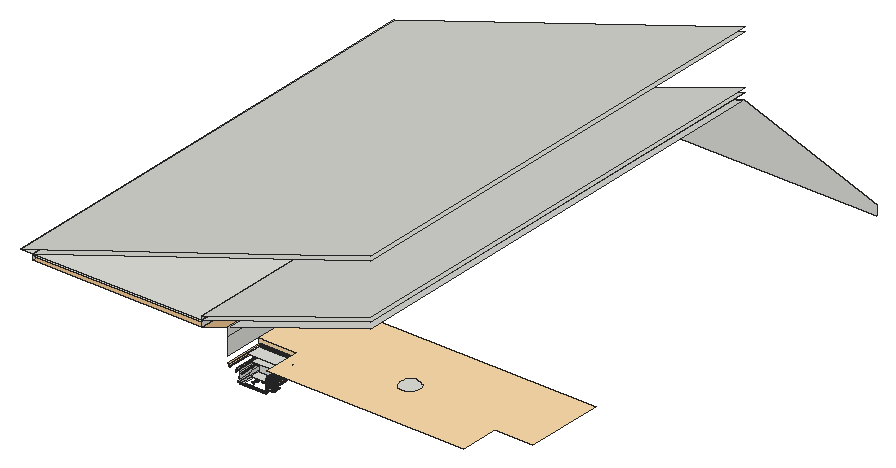
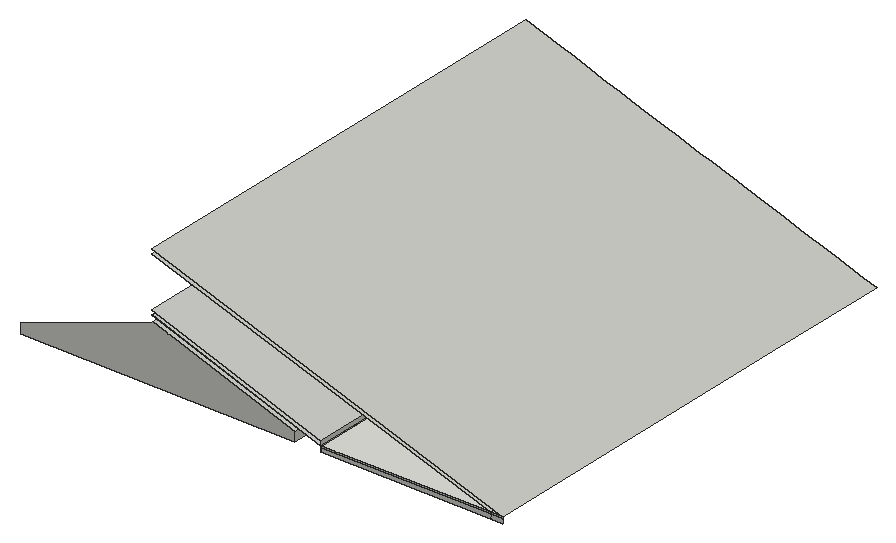
# SketchUp Ruby script. Lengths in inches.
U = 1.inch
M = Sketchup.active_model
def pt(a) = Geom::Point3d.new(a.map { |v| v * U })
def face(e, loops, mat)
  f = e.add_face(loops[0].map { |a| pt(a) })
  loops[1..].each { |l| e.add_face(l.map { |a| pt(a) }).erase! }
  f.material = f.back_material = mat if mat
  f
end
# faces: each face lists its corners as indices into pts; further lists are holes
def faces(e, pts, list, mat = nil) = list.each { |f| face(e, (f[0].is_a?(Array) ? f : [f]).map { |l| l.map { |i| pts[i] } }, mat) }
# xy, xz, yz: faces in a plane at the given z, y or x. An outline is a flat list of corners, or four numbers for a rectangle; further outlines are holes
def ring(l) = l.size == 4 ? [[l[0], l[1]], [l[2], l[1]], [l[2], l[3]], [l[0], l[3]]] : l.each_slice(2).to_a
def flat(e, list, mat, &to3) = list.each { |f| face(e, (f[0].is_a?(Array) ? f : [f]).map { |l| ring(l).map { |u, v| to3.(u, v) } }, mat) }
def xy(e, z, list, mat = nil) = flat(e, list, mat) { |x, y| [x, y, z] }
def xz(e, y, list, mat = nil) = flat(e, list, mat) { |x, z| [x, y, z] }
def yz(e, x, list, mat = nil) = flat(e, list, mat) { |y, z| [x, y, z] }
def lines(e, pts, list) = list.each { |a, b| e.add_line(pt(pts[a]), pt(pts[b])) }
# prism: a flat outline (further loops are holes) pulled along v
def prism(e, loops, v, mat = nil)
  f = face(e, loops, mat); d = Geom::Vector3d.new(v.map { |x| x * U })
  f.pushpull(f.normal.samedirection?(d) ? d.length : -d.length)
end
def box(e, o, s, mat = nil) = prism(e, [[o, [o[0] + s[0], o[1], o[2]], [o[0] + s[0], o[1] + s[1], o[2]], [o[0], o[1] + s[1], o[2]]]], [0, 0, s[2]], mat)
def at(x, y, z, deg = 0) = Geom::Transformation.translation(pt([x, y, z])) * Geom::Transformation.rotation(ORIGIN, Z_AXIS, deg.degrees)
def axes(o, x, y, z) = Geom::Transformation.new([*x, 0, *y, 0, *z, 0, *pt(o).to_a, 1])
def part(name) = M.definitions.add(name)
# library, detail: a bought-in or finely detailed component or shape, given as its bounding box
def library(name, o, s) = part(name).tap { |d| box(d.entities, o, s) }
def detail(e, o, s) = box(e.add_group.entities, o, s)
def put(e, d, t, mat = nil) = e.add_instance(d, t).tap { |i| i.material = mat if mat }
def group(e, t, mat = nil) = e.add_group.tap { |g| g.transformation = t; g.material = mat if mat }.entities
root = M.entities
M.materials.add("[0033_NavajoWhite]").color = [255, 222, 173]
M.materials.add("[0036_BurlyWood]").color = [222, 184, 135]
xy(root,94.95,[[[110.21,8.1,123.2,21.09],[111,9.67,122.41,19.51]]])
xy(root,95.99,[[110.21,14.59,123.2,21.09]])
xy(root,95.99,[[[109.69,7.58,123.72,21.61],[109.86,7.74,123.55,21.44]]],"[0033_NavajoWhite]")
xy(root,102.72,[[109.03,22.27,108.83,22.47,124.58,22.47,124.38,22.27]])
xy(root,102.72,[[108.83,22.47,108.04,23.25,125.37,23.25,124.58,22.47]],"[0033_NavajoWhite]")
xy(root,102.86,[[111,14.59,122.41,19.51]])
xy(root,105.42,[[108.83,14.59,124.58,22.47]])
xy(root,108.125,[[178.61,26.68,177.27,26.85,176.02,27.37,174.95,28.2,174.12,29.27,173.6,30.52,173.43,31.86,173.6,33.21,174.12,34.46,174.95,35.53,176.02,36.36,177.27,36.875,178.61,37.05,179.96,36.875,181.21,36.36,182.28,35.53,183.11,34.46,183.625,33.21,183.8,31.86,183.625,30.52,183.11,29.27,182.28,28.2,181.21,27.37,179.96,26.85]])
xy(root,108.125,[[[126.55,4.75,126.55,24.44,106.86,24.44,106.86,64.75,247.8,64.75,247.8,24.44,228.12,24.44,228.12,4.75],[178.61,26.68,179.96,26.85,181.21,27.37,182.28,28.2,183.11,29.27,183.625,30.52,183.8,31.86,183.625,33.21,183.11,34.46,182.28,35.53,181.21,36.36,179.96,36.875,178.61,37.05,177.27,36.875,176.02,36.36,174.95,35.53,174.12,34.46,173.6,33.21,173.43,31.86,173.6,30.52,174.12,29.27,174.95,28.2,176.02,27.37,177.27,26.85]]],"[0033_NavajoWhite]")
xy(root,117,[[6.32,4.75,93.16,64.75],[93.16,4.75,93.71,64.75]],"[0036_BurlyWood]")
xy(root,119,[[6.32,4.75,93.16,244.75]])
xy(root,120,[[0,4.75,6.32,64.75],[6.32,4.75,93.16,244.75],[0,64.75,6.32,244.75]])
xz(root,19.51,[[111,94.95,122.41,102.86]])
xz(root,21.09,[[110.21,94.95,123.2,95.1],[110.21,95.1,123.2,95.99],[110.21,95.99,123.2,97.5625],[110.21,97.5625,123.2,99.87],[110.21,99.87,123.2,100.56],
  [110.21,100.56,123.2,101.46]])
xz(root,21.61,[[109.69,95.99,123.72,96.66]])
xz(root,22.47,[[108.83,102.72,124.58,105.42]])
xz(root,24.44,[[106.86,105.42,126.55,108.125]],"[0033_NavajoWhite]")
xz(root,64.75,[[155.99,93.75,191.99,96],[93.71,117,106.86,117,106.86,121.52]])
xz(root,244.75,[[0,117,6.32,119],[6.32,117,93.16,119],[106.86,117,106.86,121.52,179.96,146.625,247.8,122.125,247.8,117],[0,119,6.32,120],[6.32,119,93.16,120]])
yz(root,6.32,[[4.75,117,64.75,119],[4.75,119,64.75,120],[64.75,119,244.75,120]])
yz(root,93.16,[[4.75,117,244.75,119],[4.75,119,244.75,119.98],[4.75,119.98,244.75,120],[4.75,120,244.75,122.1]])
yz(root,106.86,[[4.75,108.125,64.75,117],[4.75,117,64.75,121.52],[64.75,117,244.75,121.52]])
yz(root,109.69,[[7.58,95.99,21.61,96.66]])
yz(root,110.21,[[8.1,94.95,21.09,95.1],[8.1,95.1,21.09,95.99],[14.59,95.99,21.09,97.5625],[8.1,97.5625,21.09,99.87],[8.1,99.87,21.09,100.56],
  [8.1,100.56,21.09,101.46]])
yz(root,123.2,[[8.1,94.95,21.09,95.1],[8.1,95.1,21.09,95.99],[14.59,95.99,21.09,97.5625],[8.1,97.5625,21.09,99.87],[8.1,99.87,21.09,100.56],
  [8.1,100.56,21.09,101.46]])
yz(root,123.72,[[7.58,95.99,21.61,96.66]])
p = [[113.75,18.5625,92.48],[113.75,18.53,92.25],[113.5,18.5625,92.25],[113.51,18.6,92.48],[114,18.6,92.48],[114.01,18.5625,92.25],
  [116.71,18.5625,92.48],[116.71,18.53,92.25],[116.45,18.5625,92.25],[116.46,18.6,92.48],[116.95,18.6,92.48],[116.96,18.5625,92.25],
  [119.66,18.5625,92.48],[119.66,18.53,92.25],[119.4,18.5625,92.25],[119.41,18.6,92.48],[119.9,18.6,92.48],[119.91,18.5625,92.25],
  [113.26,18.66,92.25],[113.28,18.69,92.48],[114.23,18.69,92.48],[114.25,18.66,92.25],[116.21,18.66,92.25],[116.23,18.69,92.48],
  [117.18,18.69,92.48],[117.2,18.66,92.25],[119.17,18.66,92.25],[119.18,18.69,92.48],[120.13,18.69,92.48],[120.15,18.66,92.25],
  [113.06,18.82,92.25],[113.08,18.84,92.48],[114.43,18.84,92.48],[114.45,18.82,92.25],[116.01,18.82,92.25],[116.03,18.84,92.48],
  [117.38,18.84,92.48],[117.4,18.82,92.25],[118.96,18.82,92.25],[118.99,18.84,92.48],[120.33,18.84,92.48],[120.35,18.82,92.25],
  [112.9,19.02,92.25],[112.93,19.04,92.48],[114.58,19.04,92.48],[114.61,19.02,92.25],[115.85,19.02,92.25],[115.88,19.04,92.48],
  [117.53,19.04,92.48],[117.56,19.02,92.25],[118.81,19.02,92.25],[118.84,19.04,92.48],[120.48,19.04,92.48],[120.51,19.02,92.25],
  [112.8,19.26,92.25],[112.83,19.27,92.48],[114.67,19.27,92.48],[114.7,19.26,92.25],[115.76,19.26,92.25],[115.79,19.27,92.48],
  [117.625,19.27,92.48],[117.66,19.26,92.25],[118.71,19.26,92.25],[118.74,19.27,92.48],[120.58,19.27,92.48],[120.61,19.26,92.25],
  [112.77,19.51,92.25],[112.8,19.51,92.48],[114.7,19.51,92.48],[114.74,19.51,92.25],[115.72,19.51,92.25],[115.76,19.51,92.48],
  [117.66,19.51,92.48],[117.69,19.51,92.25],[118.67,19.51,92.25],[118.71,19.51,92.48],[120.61,19.51,92.48],[120.64,19.51,92.25],
  [111.92,14.84,92.74],[111.95,14.85,92.51],[111.98,14.59,92.51],[111.95,14.59,92.74],[121.46,14.85,92.51],[121.5,14.84,92.74],
  [121.46,14.59,92.74],[121.43,14.59,92.51],[111.82,15.07,92.74],[111.85,15.08,92.51],[121.5625,15.08,92.51],[121.59,15.07,92.74],
  [111.67,15.26,92.74],[111.69,15.29,92.51],[121.72,15.29,92.51],[121.74,15.26,92.74],[111.47,15.42,92.74],[111.49,15.44,92.51],
  [121.92,15.44,92.51],[121.9375,15.42,92.74],[111.24,15.51,92.74],[111.25,15.54,92.51],[122.16,15.54,92.51],[122.17,15.51,92.74],
  [111,15.54,92.74],[111,15.58,92.51],[122.41,15.54,92.74],[122.41,15.58,92.51],[111,16.59,92.74],[111.24,16.625,92.74],
  [111.25,16.59,92.51],[111,16.5625,92.51],[111.47,16.72,92.74],[111.49,16.69,92.51],[122.17,16.625,92.74],[122.16,16.59,92.51],
  [121.92,16.69,92.51],[121.9375,16.72,92.74],[122.41,16.59,92.74],[122.41,16.5625,92.51],[111.67,16.875,92.74],[111.69,16.85,92.51],
  [121.72,16.85,92.51],[121.74,16.875,92.74],[111.82,17.07,92.74],[111.85,17.05,92.51],[121.5625,17.05,92.51],[121.59,17.07,92.74],
  [111.92,17.3,92.74],[111.95,17.29,92.51],[121.46,17.29,92.51],[121.5,17.3,92.74],[111.95,17.55,92.74],[111.98,17.55,92.51],
  [121.43,17.55,92.51],[121.46,17.55,92.74],[111.92,17.79,92.74],[111.95,17.8,92.51],[121.46,17.8,92.51],[121.5,17.79,92.74],
  [111.82,18.02,92.74],[111.85,18.04,92.51],[121.5625,18.04,92.51],[121.59,18.02,92.74],[111.67,18.22,92.74],[111.69,18.24,92.51],
  [121.72,18.24,92.51],[121.74,18.22,92.74],[111.47,18.37,92.74],[111.49,18.4,92.51],[121.92,18.4,92.51],[121.9375,18.37,92.74],
  [111.24,18.46,92.74],[111.25,18.5,92.51],[122.16,18.5,92.51],[122.17,18.46,92.74],[111,18.53,92.51],[111,18.5,92.74],
  [122.41,18.53,92.51],[122.41,18.5,92.74],[113.53,18.69,92.7],[113.33,18.78,92.7],[113.75,18.66,92.7],[113.97,18.69,92.7],
  [114.18,18.78,92.7],[116.49,18.69,92.7],[116.28,18.78,92.7],[116.71,18.66,92.7],[116.93,18.69,92.7],[117.13,18.78,92.7],
  [119.4375,18.69,92.7],[119.23,18.78,92.7],[119.66,18.66,92.7],[119.88,18.69,92.7],[120.08,18.78,92.7],[113.15,18.91,92.7],
  [114.36,18.91,92.7],[116.1,18.91,92.7],[117.31,18.91,92.7],[119.06,18.91,92.7],[120.26,18.91,92.7],[113.01,19.09,92.7],
  [114.49,19.09,92.7],[115.97,19.09,92.7],[117.44,19.09,92.7],[118.92,19.09,92.7],[120.4,19.09,92.7],[112.93,19.29,92.7],
  [114.58,19.29,92.7],[115.88,19.29,92.7],[117.53,19.29,92.7],[118.84,19.29,92.7],[120.48,19.29,92.7],[112.9,19.51,92.7],
  [114.61,19.51,92.7],[115.85,19.51,92.7],[117.56,19.51,92.7],[118.81,19.51,92.7],[120.51,19.51,92.7],[111.82,14.8125,92.96],
  [111.85,14.59,92.96],[121.59,14.8125,92.96],[121.5625,14.59,92.96],[111.74,15.02,92.96],[121.68,15.02,92.96],[111.6,15.2,92.96],
  [121.8125,15.2,92.96],[111.42,15.33,92.96],[121.99,15.33,92.96],[111.22,15.42,92.96],[122.19,15.42,92.96],[111,15.44,92.96],
  [122.41,15.44,92.96],[111,16.69,92.96],[111.22,16.72,92.96],[111.42,16.81,92.96],[122.19,16.72,92.96],[121.99,16.81,92.96],
  [122.41,16.69,92.96],[111.6,16.94,92.96],[121.8125,16.94,92.96],[111.74,17.12,92.96],[121.68,17.12,92.96],[111.82,17.32,92.96],
  [121.59,17.32,92.96],[111.85,17.55,92.96],[121.5625,17.55,92.96],[111.82,17.77,92.96],[121.59,17.77,92.96],[111.74,17.97,92.96],
  [121.68,17.97,92.96],[111.6,18.15,92.96],[121.8125,18.15,92.96],[111.42,18.28,92.96],[121.99,18.28,92.96],[111.22,18.37,92.96],
  [122.19,18.37,92.96],[111,18.4,92.96],[122.41,18.4,92.96],[113.57,18.84,92.89],[113.41,18.91,92.89],[113.75,18.82,92.89],
  [113.93,18.84,92.89],[114.1,18.91,92.89],[116.53,18.84,92.89],[116.36,18.91,92.89],[116.71,18.82,92.89],[116.89,18.84,92.89],
  [117.05,18.91,92.89],[119.48,18.84,92.89],[119.3125,18.91,92.89],[119.66,18.82,92.89],[119.84,18.84,92.89],[120.01,18.91,92.89],
  [113.26,19.02,92.89],[114.25,19.02,92.89],[116.21,19.02,92.89],[117.2,19.02,92.89],[119.17,19.02,92.89],[120.15,19.02,92.89],
  [113.15,19.17,92.89],[114.36,19.17,92.89],[116.1,19.17,92.89],[117.31,19.17,92.89],[119.06,19.17,92.89],[120.26,19.17,92.89],
  [113.08,19.33,92.89],[114.43,19.33,92.89],[116.03,19.33,92.89],[117.38,19.33,92.89],[118.99,19.33,92.89],[120.33,19.33,92.89],
  [113.06,19.51,92.89],[114.45,19.51,92.89],[116.01,19.51,92.89],[117.4,19.51,92.89],[118.96,19.51,92.89],[120.35,19.51,92.89],
  [113.625,19.04,93.03],[113.51,19.09,93.03],[113.75,19.02,93.03],[113.88,19.04,93.03],[114,19.09,93.03],[116.58,19.04,93.03],
  [116.46,19.09,93.03],[116.71,19.02,93.03],[116.83,19.04,93.03],[116.95,19.09,93.03],[119.53,19.04,93.03],[119.41,19.09,93.03],
  [119.66,19.02,93.03],[119.79,19.04,93.03],[119.9,19.09,93.03],[113.41,19.17,93.03],[114.1,19.17,93.03],[116.36,19.17,93.03],
  [117.05,19.17,93.03],[119.3125,19.17,93.03],[120.01,19.17,93.03],[113.33,19.27,93.03],[114.18,19.27,93.03],[116.28,19.27,93.03],
  [117.13,19.27,93.03],[119.23,19.27,93.03],[120.08,19.27,93.03],[113.28,19.39,93.03],[114.23,19.39,93.03],[116.23,19.39,93.03],
  [117.18,19.39,93.03],[119.18,19.39,93.03],[120.13,19.39,93.03],[113.26,19.51,93.03],[114.25,19.51,93.03],[116.21,19.51,93.03],
  [117.2,19.51,93.03],[119.17,19.51,93.03],[120.15,19.51,93.03],[111.67,14.77,93.15],[111.69,14.59,93.15],[121.74,14.77,93.15],
  [121.72,14.59,93.15],[111.6,14.94,93.15],[121.8125,14.94,93.15],[111.49,15.08,93.15],[121.92,15.08,93.15],[111.35,15.2,93.15],
  [122.07,15.2,93.15],[111.18,15.26,93.15],[122.23,15.26,93.15],[111,15.29,93.15],[122.41,15.29,93.15],[111,16.85,93.15],
  [111.18,16.875,93.15],[111.35,16.94,93.15],[122.23,16.875,93.15],[122.07,16.94,93.15],[122.41,16.85,93.15],[111.49,17.05,93.15],
  [121.92,17.05,93.15],[111.6,17.2,93.15],[121.8125,17.2,93.15],[111.67,17.37,93.15],[121.74,17.37,93.15],[111.69,17.55,93.15],
  [121.72,17.55,93.15],[111.67,17.73,93.15],[121.74,17.73,93.15],[111.6,17.89,93.15],[121.8125,17.89,93.15],[111.49,18.04,93.15],
  [121.92,18.04,93.15],[111.35,18.15,93.15],[122.07,18.15,93.15],[111.18,18.22,93.15],[122.23,18.22,93.15],[111,18.24,93.15],
  [122.41,18.24,93.15],[113.6875,19.27,93.12],[113.625,19.29,93.12],[113.75,19.26,93.12],[113.82,19.27,93.12],[113.88,19.29,93.12],
  [116.64,19.27,93.12],[116.58,19.29,93.12],[116.71,19.26,93.12],[116.77,19.27,93.12],[116.83,19.29,93.12],[119.59,19.27,93.12],
  [119.53,19.29,93.12],[119.66,19.26,93.12],[119.72,19.27,93.12],[119.79,19.29,93.12],[113.57,19.33,93.12],[113.93,19.33,93.12],
  [116.53,19.33,93.12],[116.89,19.33,93.12],[119.48,19.33,93.12],[119.84,19.33,93.12],[113.53,19.39,93.12],[113.97,19.39,93.12],
  [116.49,19.39,93.12],[116.93,19.39,93.12],[119.4375,19.39,93.12],[119.88,19.39,93.12],[113.51,19.45,93.12],[114,19.45,93.12],
  [116.46,19.45,93.12],[116.95,19.45,93.12],[119.41,19.45,93.12],[119.9,19.45,93.12],[113.5,19.51,93.12],[114.01,19.51,93.12],
  [116.45,19.51,93.12],[116.96,19.51,93.12],[119.4,19.51,93.12],[119.91,19.51,93.12],[111.47,14.72,93.29],[111.49,14.59,93.29],
  [121.9375,14.72,93.29],[121.92,14.59,93.29],[111.42,14.84,93.29],[121.99,14.84,93.29],[111.35,14.94,93.29],[122.07,14.94,93.29],
  [111.24,15.02,93.29],[122.17,15.02,93.29],[111.125,15.07,93.29],[122.29,15.07,93.29],[111,15.08,93.29],[122.41,15.08,93.29],
  [111,17.05,93.29],[111.125,17.07,93.29],[122.29,17.07,93.29],[122.41,17.05,93.29],[111.24,17.12,93.29],[111.35,17.2,93.29],
  [122.17,17.12,93.29],[122.07,17.2,93.29],[111.42,17.3,93.29],[121.99,17.3,93.29],[111.47,17.42,93.29],[121.9375,17.42,93.29],
  [111.49,17.55,93.29],[121.92,17.55,93.29],[111.47,17.67,93.29],[121.9375,17.67,93.29],[111.42,17.79,93.29],[121.99,17.79,93.29],
  [111.35,17.89,93.29],[122.07,17.89,93.29],[111.24,17.97,93.29],[122.17,17.97,93.29],[111.125,18.02,93.29],[111,18.04,93.29],
  [122.29,18.02,93.29],[122.41,18.04,93.29],[113.75,19.51,93.15],[116.71,19.51,93.15],[119.66,19.51,93.15],[111.24,14.66,93.38],
  [111.25,14.59,93.38],[122.17,14.66,93.38],[122.16,14.59,93.38],[111.22,14.72,93.38],[111.18,14.77,93.38],[122.19,14.72,93.38],
  [122.23,14.77,93.38],[111.0625,14.84,93.38],[111,14.85,93.38],[111.125,14.8125,93.38],[122.29,14.8125,93.38],[122.35,14.84,93.38],
  [122.41,14.85,93.38],[111,17.29,93.38],[111.0625,17.3,93.38],[111.125,17.32,93.38],[111.18,17.37,93.38],[122.29,17.32,93.38],
  [122.23,17.37,93.38],[122.35,17.3,93.38],[122.41,17.29,93.38],[111.22,17.42,93.38],[122.19,17.42,93.38],[111.24,17.48,93.38],
  [122.17,17.48,93.38],[111.25,17.55,93.38],[122.16,17.55,93.38],[111.24,17.61,93.38],[122.17,17.61,93.38],[111.22,17.67,93.38],
  [122.19,17.67,93.38],[111.18,17.73,93.38],[111.125,17.77,93.38],[122.23,17.73,93.38],[122.29,17.77,93.38],[111.0625,17.79,93.38],
  [111,17.8,93.38],[122.35,17.79,93.38],[122.41,17.8,93.38],[111,14.59,93.41],[122.41,14.59,93.41],[111,17.55,93.41],
  [122.41,17.55,93.41],[110.2,8.09,95.25],[110.2,21.1,95.25],[110.21,21.09,95.1],[110.21,8.1,95.1],[123.2,8.1,95.1],
  [123.2,21.09,95.1],[123.21,21.1,95.25],[123.21,8.09,95.25],[110.18,8.06,95.4],[110.18,21.12,95.4],[123.23,21.12,95.4],
  [123.23,8.06,95.4],[123.26,21.15,95.53],[110.15,21.15,95.53],[123.3,21.1875,95.66],[110.11,21.1875,95.66],[123.35,21.24,95.77],
  [110.0625,21.24,95.77],[110.01,7.9,95.86],[110.01,21.29,95.86],[110.0625,7.95,95.77],[123.35,7.95,95.77],[123.4,21.29,95.86],
  [123.4,7.9,95.86],[109.95,7.84,95.93],[109.95,21.35,95.93],[123.46,21.35,95.93],[123.46,7.84,95.93],[123.52,21.41,95.98],
  [109.89,21.41,95.98],[109.86,7.74,95.99],[109.86,21.44,95.99],[109.89,7.78,95.98],[123.52,7.78,95.98],[123.55,21.44,95.99],
  [123.55,7.74,95.99],[123.84,7.45,96.68],[123.84,21.73,96.68],[123.89,21.78,96.72],[123.89,7.41,96.72],[123.79,7.51,96.66],
  [123.79,21.68,96.66],[109.57,21.73,96.68],[109.52,21.78,96.72],[109.62,21.68,96.66],[123.93,21.82,96.79],[109.48,21.82,96.79],
  [123.96,21.85,96.89],[109.45,21.85,96.89],[123.96,7.34,96.89],[123.98,21.87,96.99],[123.98,7.32,96.99],[109.43,21.87,96.99],
  [123.99,21.875,97.11],[123.99,7.31,97.11],[109.42,21.875,97.11],[123.98,21.87,97.23],[123.98,7.32,97.23],[109.43,21.87,97.23],
  [123.96,21.85,97.34],[123.96,7.34,97.34],[109.45,21.85,97.34],[123.93,21.82,97.43],[109.48,21.82,97.43],[123.89,21.78,97.5],
  [109.52,21.78,97.5],[123.89,7.41,97.5],[123.84,21.73,97.55],[123.84,7.45,97.55],[123.79,21.68,97.5625],[123.79,7.51,97.5625],
  [109.57,21.73,97.55],[109.62,21.68,97.5625],[123.69,21.58,97.74],[123.69,7.61,97.74],[109.72,21.58,97.74],[109.8125,7.7,97.93],
  [109.8125,21.49,97.93],[109.72,7.61,97.74],[123.6,21.49,97.93],[123.6,7.7,97.93],[123.52,21.4,98.14],[123.52,7.78,98.14],
  [109.9,21.4,98.14],[109.97,7.86,98.375],[109.97,21.33,98.375],[109.9,7.78,98.14],[123.44,21.33,98.375],[123.44,7.86,98.375],
  [110.04,7.92,98.62],[110.04,21.26,98.62],[123.375,21.26,98.62],[123.375,7.92,98.62],[110.09,7.98,98.875],[110.09,21.2,98.875],
  [123.32,21.2,98.875],[123.32,7.98,98.875],[110.14,8.03,99.14],[110.14,21.16,99.14],[123.27,21.16,99.14],[123.27,8.03,99.14],
  [110.18,8.0625,99.42],[110.18,21.12,99.42],[123.24,21.12,99.42],[123.24,8.0625,99.42],[123.21,21.1,99.7],[110.2,21.1,99.7],
  [110.21,8.1,99.87],[110.21,21.09,99.87],[110.2,8.09,99.7],[123.21,8.09,99.7],[123.2,21.09,99.87],[123.2,8.1,99.87],
  [108.89,6.78,100.6875],[108.89,22.41,100.6875],[108.93,22.37,100.62],[108.93,6.82,100.62],[108.98,22.32,100.57],[108.98,6.86,100.57],
  [124.43,6.86,100.57],[124.43,22.32,100.57],[124.48,22.37,100.62],[124.48,6.82,100.62],[124.52,22.41,100.6875],[124.52,6.78,100.6875],
  [124.38,6.92,100.56],[124.38,22.27,100.56],[109.03,22.27,100.56],[124.55,22.44,100.78],[124.55,6.74,100.78],[108.86,22.44,100.78],
  [124.57,22.46,100.89],[108.84,22.46,100.89],[124.57,6.73,100.89],[124.58,22.47,101.01],[124.58,6.72,101.01],[108.83,22.47,101.01],
  [124.57,22.46,101.125],[124.57,6.73,101.125],[108.84,22.46,101.125],[124.55,22.44,101.23],[108.86,22.44,101.23],[124.55,6.74,101.23],
  [124.52,22.41,101.33],[124.52,6.78,101.33],[108.89,22.41,101.33],[108.93,6.82,101.4],[108.93,22.37,101.4],[108.89,6.78,101.33],
  [124.48,22.37,101.4],[124.48,6.82,101.4],[108.98,6.86,101.44],[108.98,22.32,101.44],[124.43,22.32,101.44],[124.43,6.86,101.44],
  [124.38,22.27,101.46],[124.38,6.92,101.46],[109.03,22.27,101.46],[124.28,22.17,101.6],[124.28,7.02,101.6],[124.33,6.97,101.52],
  [124.33,22.22,101.52],[109.08,22.22,101.52],[109.13,22.17,101.6],[124.24,22.13,101.7],[124.24,7.06,101.7],[109.17,22.13,101.7],
  [124.21,22.1,101.82],[124.21,7.09,101.82],[109.2,22.1,101.82],[109.2,7.09,101.82],[109.22,7.11,101.95],[109.22,22.08,101.95],
  [124.19,22.08,101.95],[124.19,7.11,101.95],[109.23,7.11,102.09],[109.23,22.07,102.09],[124.1875,22.07,102.09],[124.1875,7.11,102.09],
  [109.22,7.11,102.23],[109.22,22.08,102.23],[124.19,22.08,102.23],[124.19,7.11,102.23],[109.2,7.09,102.36],[109.2,22.1,102.36],
  [124.21,22.1,102.36],[124.21,7.09,102.36],[124.24,22.13,102.48],[124.24,7.06,102.48],[109.17,22.13,102.48],[124.28,22.17,102.58],
  [124.28,7.02,102.58],[109.13,22.17,102.58],[124.33,22.22,102.66],[124.33,6.97,102.66],[109.08,22.22,102.66],[125.53,5.77,102.7],
  [125.53,23.41,102.7],[125.6875,23.58,102.73],[125.6875,5.61,102.73],[125.37,5.93,102.72],[125.37,23.25,102.72],[109.03,22.27,102.72],
  [124.38,22.27,102.72],[108.04,23.25,102.72],[107.88,23.41,102.7],[107.72,23.58,102.73],[107.57,23.73,102.82],[125.85,23.73,102.82],
  [125.85,5.45,102.82],[125.99,23.88,102.96],[125.99,5.3,102.96],[107.42,23.88,102.96],[107.28,5.17,103.15],[107.28,24.02,103.15],
  [107.42,5.3,102.96],[126.13,24.02,103.15],[126.13,5.17,103.15],[126.25,24.14,103.39],[126.25,5.05,103.39],[107.16,24.14,103.39],
  [126.36,24.24,103.68],[126.36,4.94,103.68],[107.05,24.24,103.68],[106.97,4.86,103.99],[106.97,24.33,103.99],[107.05,4.94,103.68],
  [126.44,24.33,103.99],[126.44,4.86,103.99],[126.51,24.39,104.33],[126.51,4.79,104.33],[106.91,24.39,104.33],[126.54,24.43,104.6875],
  [126.54,4.75,104.6875],[106.87,24.43,104.6875],[106.85,4.74,105.05],[106.85,24.45,105.05],[106.87,4.75,104.6875],[126.56,24.45,105.05],
  [126.56,4.74,105.05],[126.55,24.44,105.42],[126.55,4.75,105.42],[106.86,24.44,105.42],[106.86,4.75,121.52],[93.71,4.75,117],
  [93.71,64.75,117],[106.86,64.75,121.52],[0,4.75,120],[7.02,4.75,122.34],[14.04,4.75,124.68],[21.32,4.75,127.11],
  [27.39,4.75,129.13],[37.38,4.75,132.46],[47.5,4.75,135.83],[55.62,4.75,138.54],[66.67,4.75,142.22],[73.87,4.75,144.62],
  [84.62,4.75,148.21],[91.14,4.75,150.38],[101.33,4.75,153.78],[109.34,4.75,156.45],[117.28,4.75,159.09],[124.04,4.75,161.35],
  [131.67,4.75,163.89],[138.93,4.75,166.31],[144.16,4.75,168.05],[149.93,4.75,169.98],[155.08,4.75,171.69],[162.86,4.75,174.29],
  [180,4.75,180],[180,244.75,180],[0,244.75,120],[0,64.75,120],[6.32,4.75,120],[13.35,4.75,122.34],
  [20.37,4.75,124.68],[27.65,4.75,127.11],[33.71,4.75,129.13],[43.71,4.75,132.46],[53.83,4.75,135.83],[61.94,4.75,138.54],
  [73,4.75,142.22],[80.19,4.75,144.62],[90.94,4.75,148.21],[97.46,4.75,150.38],[107.66,4.75,153.78],[115.67,4.75,156.45],
  [123.61,4.75,159.09],[130.36,4.75,161.35],[137.99,4.75,163.89],[145.25,4.75,166.31],[150.49,4.75,168.05],[156.26,4.75,169.98],
  [161.41,4.75,171.69],[169.18,4.75,174.29],[180,4.75,177.89],[180,244.75,177.89],[6.32,244.75,120],[6.32,64.75,120],
  [179.96,4.75,149.82],[175.27,4.75,148.21],[164.84,4.75,144.62],[157.86,4.75,142.22],[147.13,4.75,138.54],[139.26,4.75,135.83],
  [129.4375,4.75,132.46],[120.04,4.75,129.23],[113.85,4.75,127.11],[106.79,4.75,124.68],[99.27,4.75,122.1],[93.16,4.75,120],
  [93.16,244.75,120],[179.96,244.75,149.82],[93.21,244.75,120],[93.21,4.75,120],[120.1,4.75,129.23],[139.33,4.75,135.83],
  [147.21,4.75,138.54],[164.92,4.75,144.62],[180,4.75,149.8],[180,244.75,149.8],[93.16,244.75,119.98],[93.16,4.75,119.98],
  [179.96,244.75,146.625],[106.86,244.75,121.52],[179.96,4.75,146.625],[180,4.75,151.93],[175.49,4.75,150.38],[169.17,4.75,148.21],
  [158.73,4.75,144.62],[151.75,4.75,142.22],[141.03,4.75,138.54],[133.15,4.75,135.83],[123.33,4.75,132.46],[113.9375,4.75,129.23],
  [107.75,4.75,127.11],[100.6875,4.75,124.68],[93.16,4.75,122.1],[93.16,244.75,122.1],[180,244.75,151.93],[123.59,14.59,96.01],
  [123.65,14.59,96.01]]
faces(root,p,[[0,1,2,3],[4,5,1,0],[6,7,8,9],[10,11,7,6],[12,13,14,15],[16,17,13,12],[3,2,18,19],[20,21,5,4],
  [9,8,22,23],[24,25,11,10],[15,14,26,27],[28,29,17,16],[19,18,30,31],[32,33,21,20],[23,22,34,35],[36,37,25,24],
  [27,26,38,39],[40,41,29,28],[31,30,42,43],[44,45,33,32],[35,34,46,47],[48,49,37,36],[39,38,50,51],[52,53,41,40],
  [43,42,54,55],[56,57,45,44],[47,46,58,59],[60,61,49,48],[51,50,62,63],[64,65,53,52],[54,66,67,55],[56,68,69,57],
  [58,70,71,59],[60,72,73,61],[62,74,75,63],[64,76,77,65],[78,79,80,81],[82,83,84,85],[86,87,79,78],[88,89,83,82],
  [90,91,87,86],[92,93,89,88],[94,95,91,90],[96,97,93,92],[98,99,95,94],[100,101,97,96],[98,102,103,99],[104,101,100,105],
  [106,107,108,109],[108,107,110,111],[112,113,114,115],[112,116,117,113],[111,110,118,119],[115,114,120,121],[119,118,122,123],[121,120,124,125],
  [123,122,126,127],[125,124,128,129],[127,126,130,131],[129,128,132,133],[131,130,134,135],[133,132,136,137],[135,134,138,139],[137,136,140,141],
  [139,138,142,143],[141,140,144,145],[143,142,146,147],[145,144,148,149],[147,146,150,151],[149,148,152,153],[154,151,150,155],[152,156,157,153],
  [158,3,19,159],[160,0,3,158],[161,4,0,160],[162,20,4,161],[163,9,23,164],[165,6,9,163],[166,10,6,165],[167,24,10,166],
  [168,15,27,169],[170,12,15,168],[171,16,12,170],[172,28,16,171],[159,19,31,173],[174,32,20,162],[164,23,35,175],[176,36,24,167],
  [169,27,39,177],[178,40,28,172],[173,31,43,179],[180,44,32,174],[175,35,47,181],[182,48,36,176],[177,39,51,183],[184,52,40,178],
  [179,43,55,185],[186,56,44,180],[181,47,59,187],[188,60,48,182],[183,51,63,189],[190,64,52,184],[55,67,191,185],[186,192,68,56],
  [59,71,193,187],[188,194,72,60],[63,75,195,189],[190,196,76,64],[197,78,81,198],[83,199,200,84],[201,86,78,197],[89,202,199,83],
  [203,90,86,201],[93,204,202,89],[205,94,90,203],[97,206,204,93],[207,98,94,205],[101,208,206,97],[207,209,102,98],[210,208,101,104],
  [211,212,107,106],[107,212,213,110],[214,112,115,215],[214,216,116,112],[110,213,217,118],[215,115,121,218],[118,217,219,122],[218,121,125,220],
  [122,219,221,126],[220,125,129,222],[126,221,223,130],[222,129,133,224],[130,223,225,134],[224,133,137,226],[134,225,227,138],[226,137,141,228],
  [138,227,229,142],[228,141,145,230],[142,229,231,146],[230,145,149,232],[146,231,233,150],[232,149,153,234],[155,150,233,235],[153,157,236,234],
  [237,158,159,238],[239,160,158,237],[240,161,160,239],[241,162,161,240],[242,163,164,243],[244,165,163,242],[245,166,165,244],[246,167,166,245],
  [247,168,169,248],[249,170,168,247],[250,171,170,249],[251,172,171,250],[238,159,173,252],[253,174,162,241],[243,164,175,254],[255,176,167,246],
  [248,169,177,256],[257,178,172,251],[252,173,179,258],[259,180,174,253],[254,175,181,260],[261,182,176,255],[256,177,183,262],[263,184,178,257],
  [258,179,185,264],[265,186,180,259],[260,181,187,266],[267,188,182,261],[262,183,189,268],[269,190,184,263],[185,191,270,264],[265,271,192,186],
  [187,193,272,266],[267,273,194,188],[189,195,274,268],[269,275,196,190],[276,237,238,277],[278,239,237,276],[279,240,239,278],[280,241,240,279],
  [281,242,243,282],[283,244,242,281],[284,245,244,283],[285,246,245,284],[286,247,248,287],[288,249,247,286],[289,250,249,288],[290,251,250,289],
  [277,238,252,291],[292,253,241,280],[282,243,254,293],[294,255,246,285],[287,248,256,295],[296,257,251,290],[291,252,258,297],[298,259,253,292],
  [293,254,260,299],[300,261,255,294],[295,256,262,301],[302,263,257,296],[297,258,264,303],[304,265,259,298],[299,260,266,305],[306,267,261,300],
  [301,262,268,307],[308,269,263,302],[264,270,309,303],[304,310,271,265],[266,272,311,305],[306,312,273,267],[268,274,313,307],[308,314,275,269],
  [315,197,198,316],[199,317,318,200],[319,201,197,315],[202,320,317,199],[321,203,201,319],[204,322,320,202],[323,205,203,321],[206,324,322,204],
  [325,207,205,323],[208,326,324,206],[325,327,209,207],[328,326,208,210],[329,330,212,211],[212,330,331,213],[332,214,215,333],[332,334,216,214],
  [213,331,335,217],[333,215,218,336],[217,335,337,219],[336,218,220,338],[219,337,339,221],[338,220,222,340],[221,339,341,223],[340,222,224,342],
  [223,341,343,225],[342,224,226,344],[225,343,345,227],[344,226,228,346],[227,345,347,229],[346,228,230,348],[229,347,349,231],[348,230,232,350],
  [231,349,351,233],[350,232,234,352],[235,233,351,353],[234,236,354,352],[355,276,277,356],[357,278,276,355],[358,279,278,357],[359,280,279,358],
  [360,281,282,361],[362,283,281,360],[363,284,283,362],[364,285,284,363],[365,286,287,366],[367,288,286,365],[368,289,288,367],[369,290,289,368],
  [356,277,291,370],[371,292,280,359],[361,282,293,372],[373,294,285,364],[366,287,295,374],[375,296,290,369],[370,291,297,376],[377,298,292,371],
  [372,293,299,378],[379,300,294,373],[374,295,301,380],[381,302,296,375],[376,297,303,382],[383,304,298,377],[378,299,305,384],[385,306,300,379],
  [380,301,307,386],[387,308,302,381],[303,309,388,382],[383,389,310,304],[305,311,390,384],[385,391,312,306],[307,313,392,386],[387,393,314,308],
  [394,315,316,395],[317,396,397,318],[398,319,315,394],[320,399,396,317],[400,321,319,398],[322,401,399,320],[402,323,321,400],[324,403,401,322],
  [404,325,323,402],[326,405,403,324],[404,406,327,325],[407,405,326,328],[408,409,330,329],[410,411,334,332],[330,409,412,331],[331,412,413,335],
  [414,333,336,415],[410,332,333,414],[335,413,416,337],[415,336,338,417],[337,416,418,339],[417,338,340,419],[339,418,420,341],[419,340,342,421],
  [341,420,422,343],[421,342,344,423],[343,422,424,345],[423,344,346,425],[345,424,426,347],[425,346,348,427],[347,426,428,349],[427,348,350,429],
  [353,351,430,431],[349,428,430,351],[429,350,352,432],[352,354,433,432],[434,370,376],[434,355,356],[434,356,370],[434,357,355],
  [434,358,357],[434,359,358],[434,371,359],[434,377,371],[435,361,372],[435,372,378],[435,362,360],[435,360,361],
  [435,363,362],[435,364,363],[435,373,364],[435,379,373],[436,374,380],[436,365,366],[436,366,374],[436,367,365],
  [436,368,367],[436,369,368],[436,375,369],[436,381,375],[434,376,382],[382,388,434],[434,383,377],[383,434,389],
  [435,378,384],[384,390,435],[435,385,379],[385,435,391],[436,380,386],[386,392,436],[436,387,381],[387,436,393],
  [437,394,395,438],[396,439,440,397],[441,398,394,437],[442,400,398,441],[399,443,439,396],[401,444,443,399],[445,446,406,404],[447,402,400,442],
  [445,404,402,447],[403,448,444,401],[405,449,448,403],[450,449,405,407],[451,452,409,408],[409,452,453,412],[412,453,454,413],[455,414,415,456],
  [457,410,414,455],[457,458,411,410],[413,454,459,416],[456,415,417,460],[416,459,461,418],[460,417,419,462],[418,461,463,420],[462,419,421,464],
  [420,463,465,422],[464,421,423,466],[422,465,467,424],[466,423,425,468],[426,469,470,428],[424,467,469,426],[468,425,427,471],[471,427,429,472],
  [431,430,473,474],[428,470,473,430],[472,429,432,475],[432,433,476,475],[477,437,438],[477,441,437],[477,442,441],[477,447,442],
  [477,445,447],[445,477,446],[439,478,440],[443,478,439],[444,478,443],[448,478,444],[449,478,448],[478,449,450],
  [479,452,451],[452,479,453],[453,479,454],[480,455,456],[457,480,458],[480,457,455],[454,479,459],[459,479,461],
  [480,456,460],[480,460,462],[461,479,463],[463,479,465],[465,479,467],[467,479,469],[469,479,470],[470,479,473],
  [474,473,479],[480,462,464],[480,464,466],[480,466,468],[480,468,471],[480,471,472],[480,472,475],[475,476,480],
  [639,640,641,642],[638,643,642,636],[643,644,639,642],[645,646,640,639],[644,647,645,639],[648,649,646,645],[647,650,648,645],[650,651,652,653],
  [654,655,649,648],[650,653,654,648],[653,652,656,657],[658,659,655,654],[653,657,658,654],[657,656,660,661],[662,663,659,658],[657,661,662,658],
  [661,660,664,665],[666,667,663,662],[661,665,666,662],[668,669,667,666],[665,670,668,666],[671,672,669,668],[670,673,671,668],[674,675,672,671],
  [673,676,674,671],[676,683,684,674],[728,729,730,731,732,733,734,735,736,737,738,739,740,741,742,743,744,745,746,747,748,749,750,751,752,753],[754,755,756,757,758,759,760,761,762,763,764,765,766,767,768,769,770,771,772,773,774,775,776,777,778,779],[780,781,782,783,784,785,786,787,788,789,790,791,792,793],[794,795,796,797,798,799,800,801],[802,803,795,794],[804,805,727,724,806],
  [807,808,809,810,811,812,813,814,815,816,817,818,819,820]])
faces(root,p,[[481,482,483,484],[485,486,487,488],[487,486,483,482],[489,490,482,481],[488,487,491,492],[491,487,482,490],[493,491,490,494],[495,493,494,496],
  [497,495,496,498],[499,500,498,501],[502,497,503,504],[503,497,498,500],[505,506,500,499],[504,503,507,508],[509,507,506,510],[507,503,500,506],
  [511,512,510,513],[514,509,515,516],[515,509,510,512],[517,518,519,520],[521,522,518,517],[519,518,523,524],[518,522,525,523],[526,519,524,527],
  [528,526,527,529],[530,528,531,532],[531,528,529,533],[532,531,534,535],[534,531,533,536],[535,534,537,538],[537,534,536,539],[538,537,540,541],
  [540,537,539,542],[543,540,542,544],[545,543,544,546],[547,545,548,549],[549,548,550,551],[548,545,546,552],[550,548,552,553],[551,550,554,555],
  [554,550,553,556],[557,558,556,559],[555,554,560,561],[560,554,556,558],[561,560,562,563],[562,560,558,564],[565,566,564,567],[563,562,568,569],
  [568,562,564,566],[570,571,566,565],[569,568,572,573],[572,568,566,571],[574,575,571,570],[573,572,576,577],[576,572,571,575],[578,579,575,574],
  [577,576,580,581],[580,576,575,579],[582,583,579,578],[581,580,584,585],[584,580,579,583],[586,584,583,587],[588,589,587,590],[591,586,592,593],
  [592,586,587,589],[594,595,596,597],[597,596,598,599],[600,601,602,603],[603,602,604,605],[606,607,601,600],[602,601,598,596],[601,607,608,598],
  [604,602,596,595],[605,604,609,610],[609,604,595,611],[612,609,611,613],[614,612,615,616],[615,612,613,617],[615,618,619,616],[618,615,617,620],
  [621,618,620,622],[623,621,624,625],[624,621,622,626],[627,628,626,629],[624,630,631,625],[630,624,626,628],[632,633,628,627],[631,630,634,635],
  [635,634,636,637],[634,630,628,633],[636,634,633,638],[677,678,679,680],[681,682,678,677],[685,686,678,682],[686,687,679,678],[687,688,689,679],
  [690,689,691,692],[688,693,691,689],[694,695,693,696],[692,691,697,698],[693,695,697,691],[698,697,699,700],[695,701,699,697],[700,699,702,703],
  [701,704,702,699],[705,706,704,707],[703,702,708,709],[704,706,708,702],[709,708,710,711],[706,712,710,708],[711,710,713,714],[712,715,713,710],
  [716,717,715,718],[714,713,719,720],[715,717,719,713],[720,719,721,722],[717,723,721,719]],"[0033_NavajoWhite]")
faces(root,p,[[724,725,726,727]],"[0036_BurlyWood]")
lines(root,p,[[821,822]])
